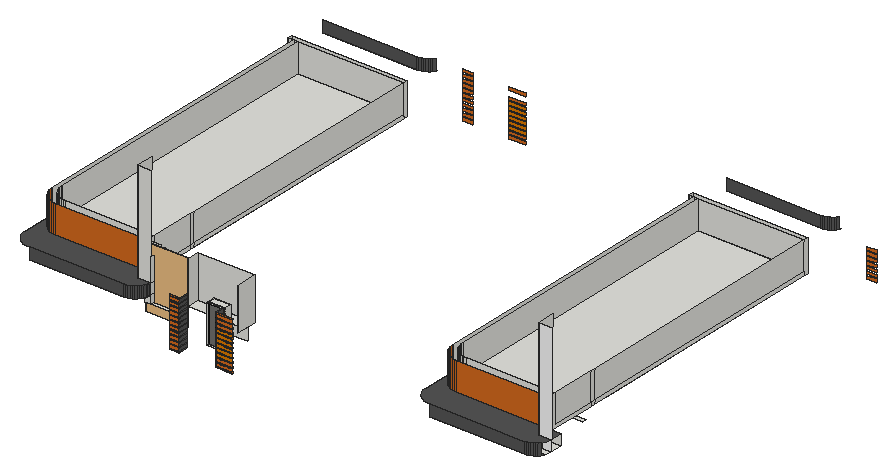
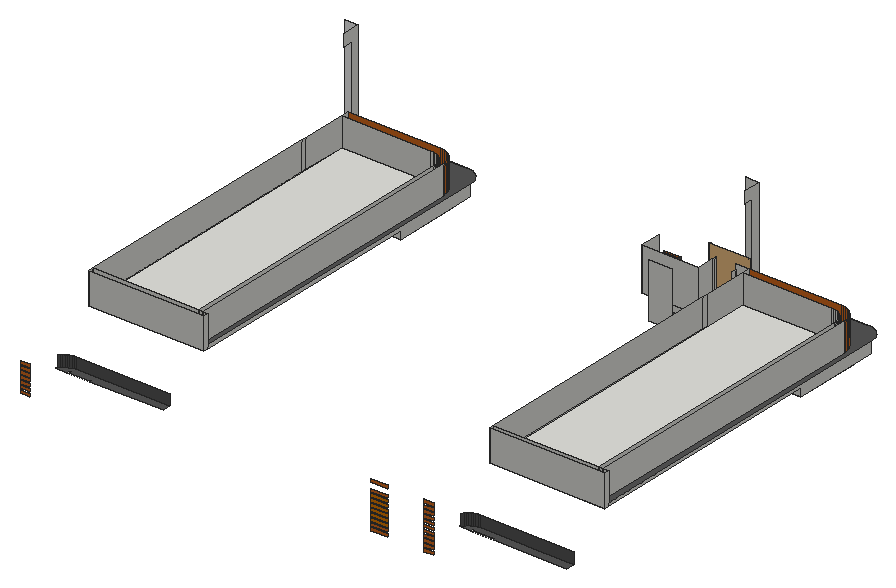
# SketchUp Ruby script. Lengths in inches.
U = 1.inch
M = Sketchup.active_model
def pt(a) = Geom::Point3d.new(a.map { |v| v * U })
def face(e, loops, mat)
  f = e.add_face(loops[0].map { |a| pt(a) })
  loops[1..].each { |l| e.add_face(l.map { |a| pt(a) }).erase! }
  f.material = f.back_material = mat if mat
  f
end
# faces: each face lists its corners as indices into pts; further lists are holes
def faces(e, pts, list, mat = nil) = list.each { |f| face(e, (f[0].is_a?(Array) ? f : [f]).map { |l| l.map { |i| pts[i] } }, mat) }
# xy, xz, yz: faces in a plane at the given z, y or x. An outline is a flat list of corners, or four numbers for a rectangle; further outlines are holes
def ring(l) = l.size == 4 ? [[l[0], l[1]], [l[2], l[1]], [l[2], l[3]], [l[0], l[3]]] : l.each_slice(2).to_a
def flat(e, list, mat, &to3) = list.each { |f| face(e, (f[0].is_a?(Array) ? f : [f]).map { |l| ring(l).map { |u, v| to3.(u, v) } }, mat) }
def xy(e, z, list, mat = nil) = flat(e, list, mat) { |x, y| [x, y, z] }
def xz(e, y, list, mat = nil) = flat(e, list, mat) { |x, z| [x, y, z] }
def yz(e, x, list, mat = nil) = flat(e, list, mat) { |y, z| [x, y, z] }
def lines(e, pts, list) = list.each { |a, b| e.add_line(pt(pts[a]), pt(pts[b])) }
# prism: a flat outline (further loops are holes) pulled along v
def prism(e, loops, v, mat = nil)
  f = face(e, loops, mat); d = Geom::Vector3d.new(v.map { |x| x * U })
  f.pushpull(f.normal.samedirection?(d) ? d.length : -d.length)
end
def box(e, o, s, mat = nil) = prism(e, [[o, [o[0] + s[0], o[1], o[2]], [o[0] + s[0], o[1] + s[1], o[2]], [o[0], o[1] + s[1], o[2]]]], [0, 0, s[2]], mat)
def at(x, y, z, deg = 0) = Geom::Transformation.translation(pt([x, y, z])) * Geom::Transformation.rotation(ORIGIN, Z_AXIS, deg.degrees)
def axes(o, x, y, z) = Geom::Transformation.new([*x, 0, *y, 0, *z, 0, *pt(o).to_a, 1])
def part(name) = M.definitions.add(name)
# library, detail: a bought-in or finely detailed component or shape, given as its bounding box
def library(name, o, s) = part(name).tap { |d| box(d.entities, o, s) }
def detail(e, o, s) = box(e.add_group.entities, o, s)
def put(e, d, t, mat = nil) = e.add_instance(d, t).tap { |i| i.material = mat if mat }
def group(e, t, mat = nil) = e.add_group.tap { |g| g.transformation = t; g.material = mat if mat }.entities
root = M.entities
M.materials.add("[0039_DarkOrange]").color = [219, 120, 0]
M.materials.add("[0041_Chocolate]").color = [210, 105, 30]
M.materials.add("[0129_WhiteSmoke]").color = [245, 245, 245]
M.materials.add("[Color M06]").color = [84, 84, 84]
M.materials.add("[Translucent Glass Gray]").color = [0, 0, 0]
M.materials["[Translucent Glass Gray]"].alpha = 0.5
c1 = library("1",[3.97,34.78,0],[101.43,33.99,0.79])
xy(root,180.58,[[897.21,280.47,912.6,281.47],[972.17,280.47,998.64,281.47]],"[0041_Chocolate]")
xy(root,182.6875,[[897.21,280.47,912.6,281.47],[972.17,280.47,998.64,281.47]],"[0041_Chocolate]")
xy(root,187.64,[[897.21,280.47,912.6,281.47],[972.17,280.47,998.64,281.47]],"[0041_Chocolate]")
xy(root,189.75,[[897.21,280.47,912.6,281.47],[972.17,280.47,998.64,281.47]],"[0041_Chocolate]")
xy(root,194.7,[[897.21,280.47,912.6,281.47],[972.17,280.47,998.64,281.47]],"[0041_Chocolate]")
xy(root,196.8125,[[972.17,280.47,998.64,281.47]],"[0039_DarkOrange]")
xy(root,196.8125,[[897.21,280.47,912.6,281.47]],"[0041_Chocolate]")
xy(root,196.89,[[944.83,295.65,971.52,298.33],[944.83,299.23,971.52,310.9]])
xy(root,201.77,[[972.17,280.47,998.64,281.47]],"[0039_DarkOrange]")
xy(root,201.77,[[897.21,280.47,912.6,281.47]],"[0041_Chocolate]")
xy(root,203.875,[[972.17,280.47,998.64,281.47]],"[0039_DarkOrange]")
xy(root,203.875,[[897.21,280.47,912.6,281.47]],"[0041_Chocolate]")
xy(root,208.83,[[972.17,280.47,998.64,281.47]],"[0039_DarkOrange]")
xy(root,208.83,[[897.21,280.47,912.6,281.47]],"[0041_Chocolate]")
xy(root,210.9375,[[972.17,280.47,998.64,281.47]],"[0039_DarkOrange]")
xy(root,210.9375,[[897.21,280.47,912.6,281.47]],"[0041_Chocolate]")
xy(root,215.89,[[972.17,280.47,998.64,281.47]],"[0039_DarkOrange]")
xy(root,215.89,[[897.21,280.47,912.6,281.47]],"[0041_Chocolate]")
xy(root,218,[[972.17,280.47,998.64,281.47]],"[0039_DarkOrange]")
xy(root,218,[[897.21,280.47,912.6,281.47]],"[0041_Chocolate]")
xy(root,222.95,[[972.17,280.47,998.64,281.47]],"[0039_DarkOrange]")
xy(root,222.95,[[897.21,280.47,912.6,281.47]],"[0041_Chocolate]")
xy(root,225.0625,[[972.17,280.47,998.64,281.47]],"[0039_DarkOrange]")
xy(root,225.0625,[[897.21,280.47,912.6,281.47]],"[0041_Chocolate]")
xy(root,226.8,[[847.59,292.45,857.24,305.58],[857.24,292.45,897.21,337.5625],[897.21,317.3125,990.02,337.5625]])
xy(root,227.53,[[777.42,395.98,824.61,403.17],[1427.92,395.98,1475.11,403.17]])
xy(root,230.02,[[972.17,280.47,998.64,281.47]],"[0039_DarkOrange]")
xy(root,230.02,[[897.21,280.47,912.6,281.47]],"[0041_Chocolate]")
xy(root,232.125,[[972.17,280.47,998.64,281.47]],"[0039_DarkOrange]")
xy(root,232.125,[[897.21,280.47,912.6,281.47]],"[0041_Chocolate]")
xy(root,237.08,[[972.17,280.47,998.64,281.47]],"[0039_DarkOrange]")
xy(root,237.08,[[897.21,280.47,912.6,281.47]],"[0041_Chocolate]")
xy(root,239.1875,[[897.21,280.47,912.6,281.47],[972.17,280.47,998.64,281.47]],"[0041_Chocolate]")
xy(root,240.16,[[832.88,278.34,836,281.47],[1483.38,278.34,1486.5,281.47],[833.13,281.47,834.37,281.55,835.6,281.79,836,281.93,836,281.47],[836,281.47,836,281.93,836.78,282.19,837.89,282.74,838.93,283.4375,839.87,284.26,840.69,285.2,841.38,286.23,841.9375,287.35,842.34,288.53,842.58,289.76,842.66,291,836,291,836,292.45,856.38,292.45,856.38,291,856.18,287.97,855.59,284.98,854.61,282.1,854.29,281.47],[854.29,281.47,857.24,281.47,857.24,291,856.38,291,856.18,287.97,855.59,284.98,854.61,282.1],
  [1483.63,281.47,1484.87,281.55,1486.1,281.79,1486.5,281.93,1486.5,281.47],[1486.5,281.47,1486.5,281.93,1487.28,282.19,1488.39,282.74,1489.43,283.4375,1490.37,284.26,1491.19,285.2,1491.88,286.23,1492.4375,287.35,1492.84,288.53,1493.08,289.76,1493.16,291,1486.5,291,1486.5,292.45,1506.88,292.45,1506.88,291,1506.68,287.97,1506.09,284.98,1505.11,282.1,1504.79,281.47],[836,281.93,836.78,282.19,837.89,282.74,838.93,283.4375,839.87,284.26,840.69,285.2,841.38,286.23,841.9375,287.35,842.34,288.53,842.58,289.76,842.66,291,836,291],[1486.5,281.93,1487.28,282.19,1488.39,282.74,1489.43,283.4375,1490.37,284.26,1491.19,285.2,1491.88,286.23,1492.4375,287.35,1492.84,288.53,1493.08,289.76,1493.16,291,1486.5,291],[856.38,291,857.24,292.45],
  [836,292.45,856.38,312.8125],[856.38,292.45,857.24,312.8125],[1486.5,292.45,1506.88,312.8125],[756.19,969.24,759.32,972.36],[1411.69,969.24,1414.82,972.36]])
xy(root,240.16,[[679.54,267.75,679.54,281.47,799,281.47,799,278.34,802.13,278.34,802.13,281.47,803.25,281.47,803.25,278.34,806.38,278.34,806.38,281.47,807.5,281.47,807.5,278.34,810.63,278.34,810.63,281.47,811.75,281.47,811.75,278.34,814.88,278.34,814.88,281.47,815.94,281.47,815.94,278.34,819.07,278.34,819.07,281.47,820.13,281.47,820.13,278.34,823.25,278.34,823.25,281.47,824.32,281.47,824.32,278.34,827.44,278.34,827.44,281.47,828.5,281.47,828.5,278.34,831.63,278.34,831.63,281.47,832.88,281.47,832.88,278.34,836,278.34,836,281.47,854.29,281.47,853.26,279.375,851.57,276.85,849.57,274.56,847.28,272.55,844.75,270.86,842.03,269.52,839.15,268.54,836.16,267.95,833.13,267.75],[1330.04,267.75,1330.04,281.47,1449.5,281.47,1449.5,278.34,1452.63,278.34,1452.63,281.47,1453.75,281.47,1453.75,278.34,1456.88,278.34,1456.88,281.47,1458,281.47,1458,278.34,1461.13,278.34,1461.13,281.47,1462.25,281.47,1462.25,278.34,1465.38,278.34,1465.38,281.47,1466.44,281.47,1466.44,278.34,1469.57,278.34,1469.57,281.47,1470.63,281.47,1470.63,278.34,1473.75,278.34,1473.75,281.47,1474.82,281.47,1474.82,278.34,1477.94,278.34,1477.94,281.47,1479,281.47,1479,278.34,1482.13,278.34,1482.13,281.47,1483.38,281.47,1483.38,278.34,1486.5,278.34,1486.5,281.47,1504.79,281.47,1503.76,279.375,1502.07,276.85,1500.07,274.56,1497.78,272.55,1495.25,270.86,1492.53,269.52,1489.65,268.54,1486.66,267.95,1483.63,267.75],[648.9,333.33,662.61,439.98],[1299.4,333.33,1313.11,439.98],[602.85,958.64,602.85,972.36,722.32,972.36,722.32,969.24,725.44,969.24,725.44,972.36,726.57,972.36,726.57,969.24,729.69,969.24,729.69,972.36,730.82,972.36,730.82,969.24,733.94,969.24,733.94,972.36,735.07,972.36,735.07,969.24,738.19,969.24,738.19,972.36,739.25,972.36,739.25,969.24,742.38,969.24,742.38,972.36,743.44,972.36,743.44,969.24,746.57,969.24,746.57,972.36,747.63,972.36,747.63,969.24,750.75,969.24,750.75,972.36,751.82,972.36,751.82,969.24,754.94,969.24,754.94,972.36,756.19,972.36,756.19,969.24,759.32,969.24,759.32,972.36,777.61,972.36,776.58,970.27,774.89,967.74,772.88,965.45,770.59,963.45,768.07,961.76,765.34,960.41,762.46,959.4375,759.48,958.84,756.44,958.64],
  [1258.35,958.64,1258.35,972.36,1377.82,972.36,1377.82,969.24,1380.94,969.24,1380.94,972.36,1382.07,972.36,1382.07,969.24,1385.19,969.24,1385.19,972.36,1386.32,972.36,1386.32,969.24,1389.44,969.24,1389.44,972.36,1390.57,972.36,1390.57,969.24,1393.69,969.24,1393.69,972.36,1394.75,972.36,1394.75,969.24,1397.88,969.24,1397.88,972.36,1398.94,972.36,1398.94,969.24,1402.07,969.24,1402.07,972.36,1403.13,972.36,1403.13,969.24,1406.25,969.24,1406.25,972.36,1407.32,972.36,1407.32,969.24,1410.44,969.24,1410.44,972.36,1411.69,972.36,1411.69,969.24,1414.82,969.24,1414.82,972.36,1433.11,972.36,1432.08,970.27,1430.39,967.74,1428.38,965.45,1426.09,963.45,1423.57,961.76,1420.84,960.41,1417.96,959.4375,1414.98,958.84,1411.94,958.64]],"[Color M06]")
xy(root,244.14,[[897.21,280.47,912.6,281.47],[972.17,280.47,998.64,281.47]],"[0041_Chocolate]")
xy(root,246.25,[[897.21,280.47,912.6,281.47],[972.17,280.47,998.64,281.47]],"[0041_Chocolate]")
xy(root,251.2,[[897.21,280.47,912.6,281.47],[972.17,280.47,998.64,281.47]],"[0041_Chocolate]")
xy(root,252.47,[[679.54,281.47,677.33,281.61,675.16,282.04,673.06,282.75,671.07,283.73,669.23,284.96,667.57,286.42,666.11,288.09,664.88,289.93,663.9,291.91,663.1875,294.01,662.76,296.18,662.61,298.39,662.61,439.98,765.68,439.98,765.68,395.98,836,395.98,836,291,842.66,291,842.58,289.76,842.34,288.53,841.9375,287.35,841.38,286.23,840.69,285.2,839.87,284.26,838.93,283.4375,837.89,282.74,836.78,282.19,835.6,281.79,834.37,281.55,833.13,281.47],[1330.04,281.47,1327.83,281.61,1325.66,282.04,1323.56,282.75,1321.57,283.73,1319.73,284.96,1318.07,286.42,1316.61,288.09,1315.38,289.93,1314.4,291.91,1313.6875,294.01,1313.26,296.18,1313.11,298.39,1313.11,439.98,1416.18,439.98,1416.18,395.98,1486.5,395.98,1486.5,291,1493.16,291,1493.08,289.76,1492.84,288.53,1492.4375,287.35,1491.88,286.23,1491.19,285.2,1490.37,284.26,1489.43,283.4375,1488.39,282.74,1487.28,282.19,1486.1,281.79,1484.87,281.55,1483.63,281.47],[[765.68,395.98,836,395.98,836,403.17,783.26,403.17,783.26,439.98,836,439.98,836,830.91,648.9,830.91,648.9,439.98,765.68,439.98],[654.4,445.49,830.5,825.41]],[[1416.18,395.98,1486.5,395.98,1486.5,403.17,1433.76,403.17,1433.76,439.98,1486.5,439.98,1486.5,830.91,1299.4,830.91,1299.4,439.98,1416.18,439.98],[1304.9,445.49,1481,825.41]],[783.26,403.17,836,439.98],
  [1433.76,403.17,1486.5,439.98],[648.9,830.91,836,838.14],[1299.4,830.91,1486.5,838.14]])
xy(root,253.3125,[[897.21,280.47,912.6,281.47],[972.17,280.47,998.64,281.47]],"[0041_Chocolate]")
xy(root,258.13,[[856.38,292.45,857.24,312.8125],[692.24,325.34,836,325.34,836,830.91,664.22,830.91,664.22,353.36,664.46,349.7,665.18,346.11,666.36,342.64,667.98,339.35,670.01,336.3,672.43,333.55,675.1875,331.13,678.23,329.09,681.52,327.47,684.99,326.29,688.59,325.58],[1342.74,325.34,1486.5,325.34,1486.5,830.91,1314.72,830.91,1314.72,353.36,1314.96,349.7,1315.68,346.11,1316.86,342.64,1318.48,339.35,1320.51,336.3,1322.93,333.55,1325.6875,331.13,1328.73,329.09,1332.02,327.47,1335.49,326.29,1339.09,325.58]])
xy(root,258.13,[[679.54,267.75,833.13,267.75,836.16,267.95,839.15,268.54,842.03,269.52,844.75,270.86,847.28,272.55,849.57,274.56,851.57,276.85,853.26,279.375,854.61,282.1,855.59,284.98,856.18,287.97,856.38,291,856.38,312.8125,686.5,312.8125,682.71,313.0625,678.98,313.8,675.38,315.02,671.97,316.71,668.81,318.82,665.95,321.32,663.45,324.18,662.67,325.34,661.33,327.34,659.65,330.75,658.43,334.35,657.6875,338.08,657.44,341.87,657.44,830.91,648.9,830.91,648.9,298.39,649.16,294.39,649.94,290.46,651.23,286.66,653,283.07,655.23,279.74,657.87,276.72,660.88,274.08,664.22,271.85,667.8125,270.08,671.61,268.79,675.54,268.01],[1330.04,267.75,1483.63,267.75,1486.66,267.95,1489.65,268.54,1492.53,269.52,1495.25,270.86,1497.78,272.55,1500.07,274.56,1502.07,276.85,1503.76,279.375,1505.11,282.1,1506.09,284.98,1506.68,287.97,1506.88,291,1506.88,312.8125,1337,312.8125,1333.21,313.0625,1329.48,313.8,1325.88,315.02,1322.47,316.71,1319.31,318.82,1316.45,321.32,1313.95,324.18,1313.17,325.34,1311.83,327.34,1310.15,330.75,1308.93,334.35,1308.1875,338.08,1307.94,341.87,1307.94,830.91,1299.4,830.91,1299.4,298.39,1299.66,294.39,1300.44,290.46,1301.73,286.66,1303.5,283.07,1305.73,279.74,1308.37,276.72,1311.38,274.08,1314.72,271.85,1318.3125,270.08,1322.11,268.79,1326.04,268.01]],"[Color M06]")
xy(root,258.27,[[944.83,295.65,971.52,298.33],[944.83,298.33,971.52,299.23],[944.83,299.23,971.52,310.9]])
xy(root,258.27,[[897.21,280.47,913.25,281.47],[971.52,280.47,998.64,281.47]],"[0041_Chocolate]")
xz(root,267.75,[[679.54,240.16,833.13,258.13],[1330.04,240.16,1483.63,258.13]],"[Color M06]")
xz(root,280.47,[[972.17,196.8125,998.64,201.77],[972.17,203.875,998.64,208.83],[972.17,210.9375,998.64,215.89],[972.17,218,998.64,222.95],[972.17,225.0625,998.64,230.02],
  [972.17,232.125,998.64,237.08]],"[0039_DarkOrange]")
xz(root,280.47,[[897.21,182.6875,912.6,187.64],[972.17,182.6875,998.64,187.64],[897.21,189.75,912.6,194.7],[972.17,189.75,998.64,194.7],[897.21,196.8125,912.6,201.77],
  [897.21,203.875,912.6,208.83],[897.21,210.9375,912.6,215.89],[897.21,218,912.6,222.95],[897.21,225.0625,912.6,230.02],[897.21,232.125,912.6,237.08],
  [897.21,239.1875,912.6,244.14],[972.17,239.1875,998.64,244.14],[897.21,246.25,912.6,251.2],[972.17,246.25,998.64,251.2],[897.21,253.3125,912.6,253.3125,913.25,258.27,897.21,258.27],
  [972.17,253.3125,998.64,253.3125,998.64,258.27,971.52,258.27]],"[0041_Chocolate]")
xz(root,281.47,[[679.54,240.16,833.13,252.47],[1330.04,240.16,1483.63,252.47]])
xz(root,281.47,[[972.17,201.77,998.64,203.875],[972.17,208.83,998.64,210.9375],[972.17,215.89,998.64,218],[972.17,222.95,998.64,225.0625],[972.17,230.02,998.64,232.125],
  [972.17,237.08,998.64,239.1875]],"[0039_DarkOrange]")
xz(root,281.47,[[897.21,180.58,912.6,182.6875],[972.17,180.58,998.64,182.6875],[897.21,187.64,912.6,189.75],[972.17,187.64,998.64,189.75],[897.21,194.7,912.6,196.8125],
  [972.17,194.7,998.64,196.8125],[897.21,201.77,912.6,203.875],[897.21,208.83,912.6,210.9375],[897.21,215.89,912.6,218],[897.21,222.95,912.6,225.0625],
  [897.21,230.02,912.6,232.125],[897.21,237.08,912.6,239.1875],[897.21,244.14,912.6,246.25],[972.17,244.14,998.64,246.25],[897.21,251.2,912.6,253.3125],
  [972.17,251.2,998.64,253.3125],[897.21,258.27,913.25,258.27,913.53,260.375,897.21,260.375],[971.52,258.27,998.64,258.27,998.64,260.375,971.24,260.375]],"[0041_Chocolate]")
xz(root,291,[[836,240.16,842.66,252.47],[1486.5,240.16,1493.16,252.47]])
xz(root,292.45,[[847.59,226.8,857.24,240.16],[836,240.16,856.38,240.16,856.38,258.13,857.24,258.13,857.24,421.25,836,421.25],[856.38,240.16,857.24,258.13]])
xz(root,292.45,[[1486.5,240.16,1506.88,240.16,1506.88,258.13,1507.74,258.13,1507.74,421.25,1486.5,421.25]],"[0129_WhiteSmoke]")
xz(root,298.33,[[944.83,196.89,971.52,258.27]],"[Translucent Glass Gray]")
xz(root,299.23,[[944.83,196.89,971.52,258.27]])
xz(root,310.9,[[944.83,196.89,971.52,258.27]])
xz(root,312.8125,[[836,240.16,856.38,258.13],[856.38,240.16,857.24,258.13],[1486.5,240.16,1506.88,258.13],[836,258.13,857.24,304.25]])
xz(root,312.8125,[[686.5,258.13,836,304.25],[1337,258.13,1486.5,304.25]],"[0041_Chocolate]")
xz(root,325.34,[[692.24,258.13,836,304.25],[1342.74,258.13,1486.5,304.25]])
xz(root,337.5625,[[897.21,226.8,990.02,295.72]])
xz(root,341.65,[[937.58,192.35,974.45,281.26]])
xz(root,439.98,[[648.9,240.16,662.61,252.47],[1299.4,240.16,1313.11,252.47]])
xz(root,830.91,[[648.9,252.47,648.9,258.13,657.44,258.13,657.44,304.25,664.22,304.25,664.22,258.13,836,258.13,836,252.47],[1299.4,252.47,1299.4,258.13,1307.94,258.13,1307.94,304.25,1314.72,304.25,1314.72,258.13,1486.5,258.13,1486.5,252.47],[648.9,258.13,657.44,304.25],[664.22,258.13,836,304.25],[1299.4,258.13,1307.94,304.25],
  [1314.72,258.13,1486.5,304.25]])
xz(root,838.14,[[648.9,252.47,836,304.25],[1299.4,252.47,1486.5,304.25]])
xz(root,958.64,[[602.85,240.16,756.44,258.13],[1258.35,240.16,1411.94,258.13]],"[Color M06]")
xz(root,971.36,[[895.48,196.8125,921.96,201.77],[895.48,203.875,921.96,208.83],[895.48,210.9375,921.96,215.89],[895.48,218,921.96,222.95],[895.48,225.0625,921.96,230.02],
  [895.48,232.125,921.96,237.08]],"[0039_DarkOrange]")
xz(root,971.36,[[820.52,182.6875,835.91,187.64],[895.48,182.6875,921.96,187.64],[1476.02,182.6875,1491.41,187.64],[820.52,189.75,835.91,194.7],[895.48,189.75,921.96,194.7],
  [1476.02,189.75,1491.41,194.7],[820.52,196.8125,835.91,201.77],[1476.02,196.8125,1491.41,201.77],[820.52,203.875,835.91,208.83],[1476.02,203.875,1491.41,208.83],
  [820.52,210.9375,835.91,215.89],[1476.02,210.9375,1491.41,215.89],[820.52,218,835.91,222.95],[1476.02,218,1491.41,222.95],[820.52,225.0625,835.91,230.02],
  [1476.02,225.0625,1491.41,230.02],[820.52,232.125,835.91,237.08],[820.52,239.1875,835.91,244.14],[895.48,239.1875,921.96,244.14],[820.52,246.25,835.91,251.2],
  [820.52,253.3125,835.91,253.3125,836.56,258.27,820.52,258.27],[895.48,253.3125,921.96,253.3125,921.96,258.27,894.83,258.27]],"[0041_Chocolate]")
yz(root,648.9,[[298.39,240.16,298.39,258.13,830.91,258.13,830.91,252.47,439.98,252.47,439.98,240.16],[830.91,252.47,838.14,304.25]])
yz(root,657.44,[[341.87,258.13,830.91,304.25]])
yz(root,662.61,[[298.39,240.16,439.98,252.47]],"[Color M06]")
yz(root,664.22,[[353.36,258.13,830.91,304.25]])
yz(root,836,[[291,240.16,292.45,252.47],[292.45,240.16,305.58,252.47],[305.58,240.16,312.8125,252.47],[292.45,252.47,292.45,421.25,321.34,421.25,321.34,402.64,305.58,402.64,305.58,252.47],[312.8125,252.47,397.86,252.47,397.86,258.13,325.34,258.13,325.34,304.25,312.8125,304.25],
  [397.86,252.47,406.38,258.13],[406.38,252.47,830.91,258.13],[830.91,252.47,838.14,304.25],[325.34,258.13,397.86,304.25],[397.86,258.13,406.38,304.25],
  [406.38,258.13,830.91,304.25]])
yz(root,856.38,[[291,240.16,292.45,258.13],[292.45,240.16,312.8125,258.13]])
yz(root,857.24,[[292.45,226.8,305.58,240.16],[305.58,226.8,321.34,240.16],[321.34,226.8,337.5625,240.16],[292.45,240.16,305.58,258.13],[312.8125,240.16,321.34,258.13],
  [321.34,240.16,337.5625,258.13],[292.45,258.13,305.58,295.72],[305.58,258.13,312.8125,295.72],[312.8125,258.13,321.34,295.72]])
yz(root,897.21,[[302.0625,226.8,302.46,295.72],[302.46,226.8,305.58,295.72],[305.58,226.8,310.27,295.72],[310.27,226.8,337.5625,295.72]])
yz(root,912.6,[[281.47,180.58,295.65,182.6875],[280.47,182.6875,295.65,187.64],[281.47,187.64,295.65,189.75],[280.47,189.75,295.65,194.7],[281.47,194.7,295.65,196.8125],
  [280.47,196.8125,295.65,201.77],[281.47,201.77,295.65,203.875],[280.47,203.875,295.65,208.83],[281.47,208.83,295.65,210.9375],[280.47,210.9375,295.65,215.89],
  [281.47,215.89,295.65,218],[280.47,218,295.65,222.95],[281.47,222.95,295.65,225.0625],[280.47,225.0625,295.65,230.02],[281.47,230.02,295.65,232.125],
  [280.47,232.125,295.65,237.08],[281.47,237.08,295.65,239.1875],[280.47,239.1875,295.65,244.14],[281.47,244.14,295.65,246.25],[280.47,246.25,295.65,251.2],
  [281.47,251.2,295.65,253.3125]],"[Color M06]")
yz(root,944.83,[[295.65,196.89,298.33,258.27],[299.23,196.89,310.9,258.27]])
yz(root,971.52,[[295.65,196.89,298.33,258.27],[299.23,196.89,310.9,258.27]])
yz(root,972.17,[[281.47,180.58,295.65,182.6875],[280.47,182.6875,295.65,187.64],[281.47,187.64,295.65,189.75],[280.47,189.75,295.65,194.7],[281.47,194.7,295.65,196.8125],
  [280.47,196.8125,295.65,201.77],[281.47,201.77,295.65,203.875],[280.47,203.875,295.65,208.83],[281.47,208.83,295.65,210.9375],[280.47,210.9375,295.65,215.89],
  [281.47,215.89,295.65,218],[280.47,218,295.65,222.95],[281.47,222.95,295.65,225.0625],[280.47,225.0625,295.65,230.02],[281.47,230.02,295.65,232.125],
  [280.47,232.125,295.65,237.08],[281.47,237.08,295.65,239.1875],[280.47,239.1875,295.65,244.14],[281.47,244.14,295.65,246.25],[280.47,246.25,295.65,251.2],
  [281.47,251.2,295.65,253.3125]],"[Color M06]")
yz(root,990.02,[[302.0625,226.8,302.46,295.72],[302.46,226.8,337.5625,295.72]])
yz(root,1299.4,[[298.39,240.16,298.39,258.13,830.91,258.13,830.91,252.47,439.98,252.47,439.98,240.16],[830.91,252.47,838.14,304.25]])
yz(root,1307.94,[[341.87,258.13,830.91,304.25]])
yz(root,1313.11,[[298.39,240.16,439.98,252.47]],"[Color M06]")
yz(root,1314.72,[[353.36,258.13,830.91,304.25]])
yz(root,1486.5,[[291,240.16,292.45,252.47],[292.45,240.16,305.58,252.47],[305.58,240.16,312.8125,252.47],[292.45,252.47,292.45,421.25,321.34,421.25,321.34,402.64,305.58,402.64,305.58,252.47],[312.8125,252.47,397.86,252.47,397.86,258.13,325.34,258.13,325.34,304.25,312.8125,304.25],
  [397.86,252.47,406.38,258.13],[406.38,252.47,830.91,258.13],[830.91,252.47,838.14,304.25],[325.34,258.13,397.86,304.25],[397.86,258.13,406.38,304.25],
  [406.38,258.13,830.91,304.25]])
p = [[836.16,267.95,258.13],[833.13,267.75,258.13],[833.13,267.75,240.16],[836.16,267.95,240.16],[1486.66,267.95,258.13],[1483.63,267.75,258.13],
  [1483.63,267.75,240.16],[1486.66,267.95,240.16],[839.15,268.54,258.13],[839.15,268.54,240.16],[1489.65,268.54,258.13],[1489.65,268.54,240.16],
  [842.03,269.52,258.13],[842.03,269.52,240.16],[1492.53,269.52,258.13],[1492.53,269.52,240.16],[844.75,270.86,258.13],[844.75,270.86,240.16],
  [1495.25,270.86,258.13],[1495.25,270.86,240.16],[847.28,272.55,258.13],[847.28,272.55,240.16],[1497.78,272.55,258.13],[1497.78,272.55,240.16],
  [849.57,274.56,258.13],[849.57,274.56,240.16],[1500.07,274.56,258.13],[1500.07,274.56,240.16],[851.57,276.85,258.13],[851.57,276.85,240.16],
  [1502.07,276.85,258.13],[1502.07,276.85,240.16],[853.26,279.375,258.13],[853.26,279.375,240.16],[854.61,282.1,258.13],[854.29,281.47,240.16],
  [854.61,282.1,240.16],[833.13,281.47,252.47],[834.37,281.55,252.47],[834.37,281.55,240.16],[833.13,281.47,240.16],[835.6,281.79,252.47],
  [835.6,281.79,240.16],[1483.63,281.47,252.47],[1484.87,281.55,252.47],[1484.87,281.55,240.16],[1483.63,281.47,240.16],[1486.1,281.79,252.47],
  [1486.1,281.79,240.16],[836.78,282.19,252.47],[836.78,282.19,240.16],[836,281.93,240.16],[1487.28,282.19,252.47],[1487.28,282.19,240.16],
  [1486.5,281.93,240.16],[855.59,284.98,258.13],[855.59,284.98,240.16],[837.89,282.74,252.47],[837.89,282.74,240.16],[1488.39,282.74,252.47],
  [1488.39,282.74,240.16],[838.93,283.4375,252.47],[838.93,283.4375,240.16],[1489.43,283.4375,252.47],[1489.43,283.4375,240.16],[839.87,284.26,252.47],
  [839.87,284.26,240.16],[1490.37,284.26,252.47],[1490.37,284.26,240.16],[840.69,285.2,252.47],[840.69,285.2,240.16],[1491.19,285.2,252.47],
  [1491.19,285.2,240.16],[856.18,287.97,258.13],[856.18,287.97,240.16],[841.38,286.23,252.47],[841.38,286.23,240.16],[1491.88,286.23,252.47],
  [1491.88,286.23,240.16],[841.9375,287.35,252.47],[841.9375,287.35,240.16],[1492.4375,287.35,252.47],[1492.4375,287.35,240.16],[842.34,288.53,252.47],
  [842.34,288.53,240.16],[1492.84,288.53,252.47],[1492.84,288.53,240.16],[856.38,291,258.13],[856.38,291,240.16],[842.58,289.76,252.47],
  [842.58,289.76,240.16],[1493.08,289.76,252.47],[1493.08,289.76,240.16],[842.66,291,252.47],[842.66,291,240.16],[1493.16,291,252.47],
  [1493.16,291,240.16],[759.48,958.84,258.13],[756.44,958.64,258.13],[756.44,958.64,240.16],[759.48,958.84,240.16],[1414.98,958.84,258.13],
  [1411.94,958.64,258.13],[1411.94,958.64,240.16],[1414.98,958.84,240.16],[762.46,959.4375,258.13],[762.46,959.4375,240.16],[1417.96,959.4375,258.13],
  [1417.96,959.4375,240.16],[765.34,960.41,258.13],[765.34,960.41,240.16],[1420.84,960.41,258.13],[1420.84,960.41,240.16],[768.07,961.76,258.13],
  [768.07,961.76,240.16],[1423.57,961.76,258.13],[1423.57,961.76,240.16],[770.59,963.45,258.13],[770.59,963.45,240.16],[1426.09,963.45,258.13],
  [1426.09,963.45,240.16],[772.88,965.45,258.13],[772.88,965.45,240.16],[1428.38,965.45,258.13],[1428.38,965.45,240.16],[774.89,967.74,258.13],
  [774.89,967.74,240.16],[1430.39,967.74,258.13],[1430.39,967.74,240.16],[776.58,970.27,258.13],[776.58,970.27,240.16],[1432.08,970.27,258.13],
  [1432.08,970.27,240.16],[913.25,295.65,258.27],[913.25,281.47,258.27],[913.25,280.47,258.27],[912.6,280.47,253.3125],[912.6,281.47,253.3125],
  [912.6,295.65,253.3125],[972.17,295.65,253.3125],[972.17,281.47,253.3125],[972.17,280.47,253.3125],[971.52,280.47,258.27],[971.52,281.47,258.27],
  [971.52,295.65,258.27],[682.71,313.0625,258.13],[686.5,312.8125,258.13],[686.5,312.8125,304.25],[682.71,313.0625,304.25],[1333.21,313.0625,258.13],
  [1337,312.8125,258.13],[1337,312.8125,304.25],[1333.21,313.0625,304.25],[678.98,313.8,258.13],[678.98,313.8,304.25],[1329.48,313.8,258.13],
  [1329.48,313.8,304.25],[675.38,315.02,258.13],[675.38,315.02,304.25],[1325.88,315.02,258.13],[1325.88,315.02,304.25],[671.97,316.71,258.13],
  [671.97,316.71,304.25],[1322.47,316.71,258.13],[1322.47,316.71,304.25],[668.81,318.82,258.13],[668.81,318.82,304.25],[1319.31,318.82,258.13],
  [1319.31,318.82,304.25],[665.95,321.32,258.13],[665.95,321.32,304.25],[1316.45,321.32,258.13],[1316.45,321.32,304.25],[663.45,324.18,258.13],
  [664.22,323.29,304.25],[663.45,324.18,304.25],[1313.95,324.18,258.13],[1314.72,323.29,304.25],[1313.95,324.18,304.25],[662.67,325.34,258.13],
  [662.67,325.34,304.25],[1313.17,325.34,258.13],[1313.17,325.34,304.25],[661.33,327.34,258.13],[661.33,327.34,304.25],[692.24,325.34,258.13],
  [688.59,325.58,258.13],[688.59,325.58,304.25],[692.24,325.34,304.25],[1311.83,327.34,258.13],[1311.83,327.34,304.25],[1342.74,325.34,258.13],
  [1339.09,325.58,258.13],[1339.09,325.58,304.25],[1342.74,325.34,304.25],[684.99,326.29,258.13],[684.99,326.29,304.25],[1335.49,326.29,258.13],
  [1335.49,326.29,304.25],[681.52,327.47,258.13],[681.52,327.47,304.25],[1332.02,327.47,258.13],[1332.02,327.47,304.25],[659.65,330.75,258.13],
  [659.65,330.75,304.25],[1310.15,330.75,258.13],[1310.15,330.75,304.25],[678.23,329.09,258.13],[678.23,329.09,304.25],[1328.73,329.09,258.13],
  [1328.73,329.09,304.25],[675.1875,331.13,258.13],[675.1875,331.13,304.25],[1325.6875,331.13,258.13],[1325.6875,331.13,304.25],[658.43,334.35,258.13],
  [658.43,334.35,304.25],[1308.93,334.35,258.13],[1308.93,334.35,304.25],[672.43,333.55,258.13],[672.43,333.55,304.25],[1322.93,333.55,258.13],
  [1322.93,333.55,304.25],[670.01,336.3,258.13],[670.01,336.3,304.25],[1320.51,336.3,258.13],[1320.51,336.3,304.25],[657.6875,338.08,258.13],
  [657.6875,338.08,304.25],[1308.1875,338.08,258.13],[1308.1875,338.08,304.25],[667.98,339.35,258.13],[667.98,339.35,304.25],[1318.48,339.35,258.13],
  [1318.48,339.35,304.25],[657.44,341.87,258.13],[657.44,341.87,304.25],[1307.94,341.87,258.13],[1307.94,341.87,304.25],[666.36,342.64,258.13],
  [666.36,342.64,304.25],[1316.86,342.64,258.13],[1316.86,342.64,304.25],[665.18,346.11,258.13],[665.18,346.11,304.25],[1315.68,346.11,258.13],
  [1315.68,346.11,304.25],[664.46,349.7,258.13],[664.46,349.7,304.25],[1314.96,349.7,258.13],[1314.96,349.7,304.25],[664.22,353.36,258.13],
  [664.22,353.36,304.25],[1314.72,353.36,258.13],[1314.72,353.36,304.25],[913.53,281.47,260.375],[913.53,295.65,260.375],[971.24,281.47,260.375],
  [971.24,295.65,260.375],[937.58,321.34,192.35],[937.58,341.65,192.35]]
faces(root,p,[[0,1,2,3],[4,5,6,7],[8,0,3,9],[10,4,7,11],[12,8,9,13],[14,10,11,15],[16,12,13,17],[18,14,15,19],
  [20,16,17,21],[22,18,19,23],[24,20,21,25],[26,22,23,27],[28,24,25,29],[30,26,27,31],[32,28,29,33],[34,32,33,35,36],
  [55,34,36,56],[73,55,56,74],[87,73,74,88],[97,98,99,100],[101,102,103,104],[105,97,100,106],[107,101,104,108],[109,105,106,110],
  [111,107,108,112],[113,109,110,114],[115,111,112,116],[117,113,114,118],[119,115,116,120],[121,117,118,122],[123,119,120,124],[125,121,122,126],
  [127,123,124,128],[129,125,126,130],[131,127,128,132],[133,134,135,136,137,138],[139,140,141,142,143,144],[255,134,133,256],[143,257,258,144]],"[Color M06]")
faces(root,p,[[37,38,39,40],[38,41,42,39],[43,44,45,46],[44,47,48,45],[41,49,50,51,42],[47,52,53,54,48],[49,57,58,50],[52,59,60,53],
  [57,61,62,58],[59,63,64,60],[61,65,66,62],[63,67,68,64],[65,69,70,66],[67,71,72,68],[69,75,76,70],[71,77,78,72],
  [75,79,80,76],[77,81,82,78],[79,83,84,80],[81,85,86,82],[83,89,90,84],[85,91,92,86],[89,93,94,90],[91,95,96,92],
  [185,186,187,188],[191,192,193,194],[186,195,196,187],[192,197,198,193],[195,199,200,196],[197,201,202,198],[199,207,208,200],[201,209,210,202],
  [207,211,212,208],[209,213,214,210],[211,219,220,212],[213,221,222,214],[219,223,224,220],[221,225,226,222],[223,231,232,224],[225,233,234,226],
  [231,239,240,232],[233,241,242,234],[239,243,244,240],[241,245,246,242],[243,247,248,244],[245,249,250,246],[247,251,252,248],[249,253,254,250]])
faces(root,p,[[145,146,147,148],[149,150,151,152],[153,145,148,154],[155,149,152,156],[157,153,154,158],[159,155,156,160],[161,157,158,162],[163,159,160,164],
  [165,161,162,166],[167,163,164,168],[169,165,166,170],[171,167,168,172],[173,169,170,174,175],[176,171,172,177,178],[179,173,175,180],[181,176,178,182],
  [183,179,180,184],[189,181,182,190],[203,183,184,204],[205,189,190,206],[215,203,204,216],[217,205,206,218],[227,215,216,228],[229,217,218,230],
  [235,227,228,236],[237,229,230,238]],"[0041_Chocolate]")
lines(root,p,[[259,260]])
put(root,c1,axes([980.87,299.43,204.87],[0,0,1],[-2,0,0],[0,-1,0]))
